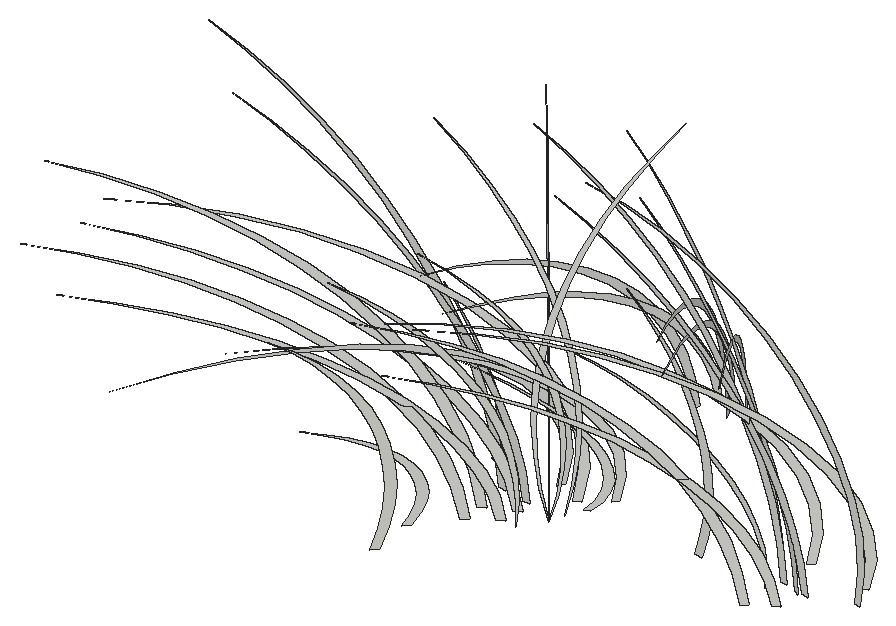
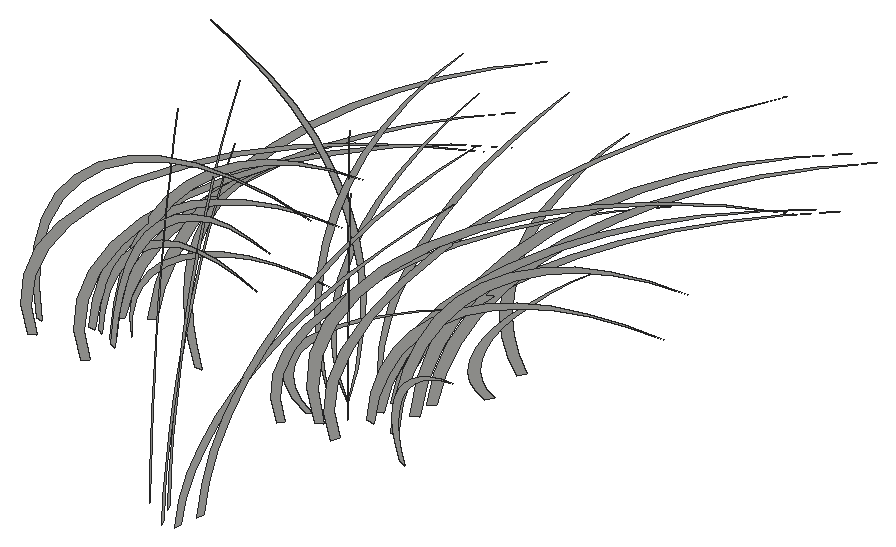
# SketchUp Ruby script. Lengths in inches.
U = 1.inch
M = Sketchup.active_model
def pt(a) = Geom::Point3d.new(a.map { |v| v * U })
def face(e, loops, mat)
  f = e.add_face(loops[0].map { |a| pt(a) })
  loops[1..].each { |l| e.add_face(l.map { |a| pt(a) }).erase! }
  f.material = f.back_material = mat if mat
  f
end
# faces: each face lists its corners as indices into pts; further lists are holes
def faces(e, pts, list, mat = nil) = list.each { |f| face(e, (f[0].is_a?(Array) ? f : [f]).map { |l| l.map { |i| pts[i] } }, mat) }
# xy, xz, yz: faces in a plane at the given z, y or x. An outline is a flat list of corners, or four numbers for a rectangle; further outlines are holes
def ring(l) = l.size == 4 ? [[l[0], l[1]], [l[2], l[1]], [l[2], l[3]], [l[0], l[3]]] : l.each_slice(2).to_a
def flat(e, list, mat, &to3) = list.each { |f| face(e, (f[0].is_a?(Array) ? f : [f]).map { |l| ring(l).map { |u, v| to3.(u, v) } }, mat) }
def xy(e, z, list, mat = nil) = flat(e, list, mat) { |x, y| [x, y, z] }
def xz(e, y, list, mat = nil) = flat(e, list, mat) { |x, z| [x, y, z] }
def yz(e, x, list, mat = nil) = flat(e, list, mat) { |y, z| [x, y, z] }
def lines(e, pts, list) = list.each { |a, b| e.add_line(pt(pts[a]), pt(pts[b])) }
# prism: a flat outline (further loops are holes) pulled along v
def prism(e, loops, v, mat = nil)
  f = face(e, loops, mat); d = Geom::Vector3d.new(v.map { |x| x * U })
  f.pushpull(f.normal.samedirection?(d) ? d.length : -d.length)
end
def box(e, o, s, mat = nil) = prism(e, [[o, [o[0] + s[0], o[1], o[2]], [o[0] + s[0], o[1] + s[1], o[2]], [o[0], o[1] + s[1], o[2]]]], [0, 0, s[2]], mat)
def at(x, y, z, deg = 0) = Geom::Transformation.translation(pt([x, y, z])) * Geom::Transformation.rotation(ORIGIN, Z_AXIS, deg.degrees)
def axes(o, x, y, z) = Geom::Transformation.new([*x, 0, *y, 0, *z, 0, *pt(o).to_a, 1])
def part(name) = M.definitions.add(name)
# library, detail: a bought-in or finely detailed component or shape, given as its bounding box
def library(name, o, s) = part(name).tap { |d| box(d.entities, o, s) }
def detail(e, o, s) = box(e.add_group.entities, o, s)
def put(e, d, t, mat = nil) = e.add_instance(d, t).tap { |i| i.material = mat if mat }
def group(e, t, mat = nil) = e.add_group.tap { |g| g.transformation = t; g.material = mat if mat }.entities
root = M.entities
g1 = group(root,at(60.55,564.61,0.02))
p = [[-20.46,3.64,18.05],[-23.54,4.19,18.53],[-20.55,3.66,17.95],[-17.67,3.15,17.15],[-14.91,2.66,16.14],[-12.33,2.2,14.93],
  [-9.93,1.77,13.53],[-7.76,1.38,11.96],[-5.84,1.04,10.23],[-4.18,0.74,8.37],[-2.8,0.5,6.39],[-1.73,0.31,4.32],
  [-0.97,0.17,2.18],[-0.53,0.09,0],[0,0,0],[-0.36,0.0625,2.23],[-1.07,0.19,4.43],[-2.125,0.38,6.55],
  [-3.51,0.625,8.57],[-5.2,0.93,10.47],[-7.1875,1.28,12.22],[-9.43,1.68,13.8],[-11.92,2.125,15.1875],[-14.61,2.6,16.37],
  [-17.46,3.11,17.33]]
faces(g1,p,[[0,1,2,3,4,5,6,7,8,9,10,11,12,13,14,15,16,17,18,19,20,21,22,23,24]])
g2 = group(root,at(60.9375,562.5,0.02))
p = [[-18.45,-9.5625,18.05],[-21.23,-11,18.53],[-18.53,-9.61,17.95],[-15.93,-8.26,17.15],[-13.45,-6.97,16.14],[-11.12,-5.76,14.93],
  [-8.96,-4.64,13.53],[-7,-3.63,11.96],[-5.26,-2.73,10.23],[-3.77,-1.95,8.37],[-2.53,-1.3125,6.39],[-1.5625,-0.81,4.32],
  [-0.875,-0.45,2.18],[-0.48,-0.25,0],[0,0,0],[-0.32,-0.17,2.23],[-0.97,-0.5,4.43],[-1.92,-0.99,6.55],
  [-3.16,-1.64,8.57],[-4.69,-2.43,10.47],[-6.48,-3.36,12.22],[-8.51,-4.41,13.8],[-10.75,-5.57,15.1875],[-13.17,-6.83,16.37],
  [-15.75,-8.16,17.33]]
faces(g2,p,[[0,1,2,3,4,5,6,7,8,9,10,11,12,13,14,15,16,17,18,19,20,21,22,23,24]])
g3 = group(root,at(60.9375,562.5,0.02))
p = [[-18.45,-9.5625,18.05],[-21.23,-11,18.53],[-18.53,-9.61,17.95],[-15.93,-8.26,17.15],[-13.45,-6.97,16.14],[-11.12,-5.76,14.93],
  [-8.96,-4.64,13.53],[-7,-3.63,11.96],[-5.26,-2.73,10.23],[-3.77,-1.95,8.37],[-2.53,-1.3125,6.39],[-1.5625,-0.81,4.32],
  [-0.875,-0.45,2.18],[-0.48,-0.25,0],[0,0,0],[-0.32,-0.17,2.23],[-0.97,-0.5,4.43],[-1.92,-0.99,6.55],
  [-3.16,-1.64,8.57],[-4.69,-2.43,10.47],[-6.48,-3.36,12.22],[-8.51,-4.41,13.8],[-10.75,-5.57,15.1875],[-13.17,-6.83,16.37],
  [-15.75,-8.16,17.33]]
faces(g3,p,[[0,1,2,3,4,5,6,7,8,9,10,11,12,13,14,15,16,17,18,19,20,21,22,23,24]])
g4 = group(root,at(62.45,564.27,0.02))
p = [[-20.46,3.64,14.56],[-23.54,4.19,14.94],[-20.55,3.66,14.48],[-17.67,3.15,13.83],[-14.91,2.66,13.02],[-12.33,2.2,12.04],
  [-9.93,1.77,10.91],[-7.76,1.38,9.64],[-5.84,1.04,8.25],[-4.18,0.74,6.75],[-2.8,0.5,5.15],[-1.73,0.31,3.49],
  [-0.97,0.17,1.76],[-0.53,0.09,0],[0,0,0],[-0.36,0.0625,1.8],[-1.07,0.19,3.57],[-2.125,0.38,5.28],
  [-3.51,0.625,6.91],[-5.2,0.93,8.44],[-7.1875,1.28,9.85],[-9.43,1.68,11.13],[-11.92,2.125,12.25],[-14.61,2.6,13.2],
  [-17.46,3.11,13.97]]
faces(g4,p,[[0,1,2,3,4,5,6,7,8,9,10,11,12,13,14,15,16,17,18,19,20,21,22,23,24]])
g5 = group(root,at(60.98,561.01,0.02))
p = [[-17.17,-11.7,15.34],[-19.76,-13.47,15.75],[-17.25,-11.76,15.26],[-14.83,-10.11,14.58],[-12.52,-8.53,13.72],[-10.35,-7.05,12.69],
  [-8.34,-5.68,11.5],[-6.52,-4.44,10.16],[-4.9,-3.34,8.7],[-3.51,-2.39,7.11],[-2.35,-1.6,5.43],[-1.45,-0.99,3.67],
  [-0.82,-0.56,1.86],[-0.45,-0.3,0],[0,0,0],[-0.3,-0.21,1.9],[-0.9,-0.61,3.76],[-1.78,-1.22,5.57],
  [-2.95,-2.01,7.28],[-4.37,-2.98,8.9],[-6.03,-4.11,10.39],[-7.92,-5.4,11.73],[-10,-6.82,12.91],[-12.26,-8.36,13.91],
  [-14.66,-9.99,14.73]]
faces(g5,p,[[0,1,2,3,4,5,6,7,8,9,10,11,12,13,14,15,16,17,18,19,20,21,22,23,24]])
g6 = group(root,at(62.65,563.39,0.02))
p = [[-18.45,-9.5625,14.56],[-21.23,-11,14.94],[-18.53,-9.61,14.48],[-15.93,-8.26,13.83],[-13.45,-6.97,13.02],[-11.12,-5.76,12.04],
  [-8.96,-4.64,10.91],[-7,-3.63,9.64],[-5.26,-2.73,8.25],[-3.77,-1.95,6.75],[-2.53,-1.3125,5.15],[-1.5625,-0.81,3.49],
  [-0.875,-0.45,1.76],[-0.48,-0.25,0],[0,0,0],[-0.32,-0.17,1.8],[-0.97,-0.5,3.57],[-1.92,-0.99,5.28],
  [-3.16,-1.64,6.91],[-4.69,-2.43,8.44],[-6.48,-3.36,9.85],[-8.51,-4.41,11.13],[-10.75,-5.57,12.25],[-13.17,-6.83,13.2],
  [-15.75,-8.16,13.97]]
faces(g6,p,[[0,1,2,3,4,5,6,7,8,9,10,11,12,13,14,15,16,17,18,19,20,21,22,23,24]])
g7 = group(root,at(62.65,563.39,0.02))
p = [[-18.45,-9.5625,14.56],[-21.23,-11,14.94],[-18.53,-9.61,14.48],[-15.93,-8.26,13.83],[-13.45,-6.97,13.02],[-11.12,-5.76,12.04],
  [-8.96,-4.64,10.91],[-7,-3.63,9.64],[-5.26,-2.73,8.25],[-3.77,-1.95,6.75],[-2.53,-1.3125,5.15],[-1.5625,-0.81,3.49],
  [-0.875,-0.45,1.76],[-0.48,-0.25,0],[0,0,0],[-0.32,-0.17,1.8],[-0.97,-0.5,3.57],[-1.92,-0.99,5.28],
  [-3.16,-1.64,6.91],[-4.69,-2.43,8.44],[-6.48,-3.36,9.85],[-8.51,-4.41,11.13],[-10.75,-5.57,12.25],[-13.17,-6.83,13.2],
  [-15.75,-8.16,13.97]]
faces(g7,p,[[0,1,2,3,4,5,6,7,8,9,10,11,12,13,14,15,16,17,18,19,20,21,22,23,24]])
g8 = group(root,at(62.58,562.1,0.02))
p = [[-17.17,-11.7,12.375],[-19.76,-13.47,12.7],[-17.25,-11.76,12.31],[-14.83,-10.11,11.76],[-12.52,-8.53,11.07],[-10.35,-7.05,10.23],
  [-8.34,-5.68,9.27],[-6.52,-4.44,8.2],[-4.9,-3.34,7.01],[-3.51,-2.39,5.74],[-2.35,-1.6,4.38],[-1.45,-0.99,2.96],
  [-0.82,-0.56,1.5],[-0.45,-0.3,0],[0,0,0],[-0.3,-0.21,1.53],[-0.9,-0.61,3.03],[-1.78,-1.22,4.49],
  [-2.95,-2.01,5.875],[-4.37,-2.98,7.18],[-6.03,-4.11,8.375],[-7.92,-5.4,9.46],[-10,-6.82,10.41],[-12.26,-8.36,11.22],
  [-14.66,-9.99,11.88]]
faces(g8,p,[[0,1,2,3,4,5,6,7,8,9,10,11,12,13,14,15,16,17,18,19,20,21,22,23,24]])
g9 = group(root,at(64.78,566.42,0.02))
p = [[-0.82,-0.43,0],[-0.36,-0.1875,0],[0,0,2.0625],[-0.15,-0.08,4.13],[-0.8,-0.42,6.16],[-1.95,-1.01,8.1],
  [-3.57,-1.85,9.91],[-5.6,-2.9,11.52],[-8.01,-4.15,12.92],[-10.74,-5.57,14.05],[-13.71,-7.1,14.9],[-16.85,-8.73,15.45],
  [-20.09,-10.41,15.67],[-23.34,-12.1,15.5625],[-20.15,-10.44,15.58],[-16.99,-8.81,15.29],[-13.9375,-7.22,14.71],[-11.06,-5.73,13.83],
  [-8.42,-4.37,12.68],[-6.09,-3.16,11.3],[-4.11,-2.13,9.7],[-2.53,-1.3125,7.9375],[-1.4,-0.72,6.04],[-0.72,-0.375,4.05],
  [-0.53,-0.27,2.02]]
faces(g9,p,[[0,1,2,3,4,5,6,7,8,9,10,11,12,13,14,15,16,17,18,19,20,21,22,23,24]])
g10 = group(root,at(59.1,566.3,0.02))
p = [[-6.53,2.99,7.88],[-5.33,2.44,7.38],[-4.26,1.95,6.83],[-3.3,1.51,6.24],[-2.48,1.14,5.62],[-1.81,0.83,4.96],
  [-1.28,0.58,4.27],[-0.9,0.41,3.57],[-0.68,0.31,2.86],[-0.61,0.28,2.13],[-0.71,0.32,1.41],[-0.96,0.4375,0.7],
  [-1.37,0.625,0],[-0.84,0.38,0],[-0.39,0.18,0.71],[-0.11,0.05,1.43],[0,0,2.17],[-0.07,0.03,2.9],
  [-0.32,0.15,3.63],[-0.74,0.34,4.34],[-1.33,0.61,5.03],[-2.08,0.95,5.69],[-2.99,1.37,6.3125],[-4.04,1.85,6.89],
  [-5.22,2.39,7.41]]
faces(g10,p,[[0,1,2,3,4,5,6,7,8,9,10,11,12,13,14,15,16,17,18,19,20,21,22,23,24]])
g11 = group(root,at(62.69,567.61,0.02))
p = [[-0.37,-0.92,0],[-0.16,-0.41,0],[0,0,1.75],[-0.07,-0.17,3.51],[-0.36,-0.9,5.24],[-0.88,-2.19,6.89],
  [-1.61,-4,8.42],[-2.53,-6.28,9.8],[-3.61,-8.99,10.98],[-4.84,-12.04,11.95],[-6.18,-15.375,12.67],[-7.6,-18.9,13.13],
  [-9.06,-22.53,13.32],[-10.53,-26.18,13.23],[-9.09,-22.6,13.25],[-7.66,-19.06,13],[-6.29,-15.63,12.5],[-4.99,-12.41,11.75],
  [-3.8,-9.45,10.78],[-2.75,-6.83,9.6],[-1.85,-4.61,8.25],[-1.14,-2.84,6.75],[-0.63,-1.57,5.13],[-0.33,-0.8125,3.44],
  [-0.24,-0.59,1.72]]
faces(g11,p,[[0,1,2,3,4,5,6,7,8,9,10,11,12,13,14,15,16,17,18,19,20,21,22,23,24]])
g12 = group(root,at(59.4375,559.42,0.02))
p = [[-3.94,-6,6.7],[-3.22,-4.9,6.27],[-2.57,-3.91,5.81],[-2,-3.04,5.31],[-1.5,-2.28,4.77],[-1.09,-1.66,4.21],
  [-0.77,-1.17,3.63],[-0.54,-0.83,3.03],[-0.41,-0.62,2.43],[-0.37,-0.5625,1.8125],[-0.43,-0.65,1.2],[-0.58,-0.88,0.59],
  [-0.83,-1.26,0],[-0.51,-0.77,0],[-0.23,-0.36,0.6],[-0.0625,-0.1,1.22],[0,0,1.84],[-0.04,-0.07,2.47],
  [-0.19,-0.29,3.09],[-0.45,-0.68,3.69],[-0.8,-1.22,4.28],[-1.26,-1.91,4.84],[-1.81,-2.75,5.37],[-2.44,-3.71,5.86],
  [-3.16,-4.8,6.3]]
faces(g12,p,[[0,1,2,3,4,5,6,7,8,9,10,11,12,13,14,15,16,17,18,19,20,21,22,23,24]])
g13 = group(root,at(59.73,556.34,0.02))
p = [[-3.94,-6,13.62],[-3.22,-4.9,12.76],[-2.57,-3.91,11.81],[-2,-3.04,10.79],[-1.5,-2.28,9.7],[-1.09,-1.66,8.57],
  [-0.77,-1.17,7.38],[-0.54,-0.83,6.17],[-0.41,-0.62,4.93],[-0.37,-0.5625,3.6875],[-0.43,-0.65,2.44],[-0.58,-0.88,1.21],
  [-0.83,-1.26,0],[-0.51,-0.77,0],[-0.23,-0.36,1.22],[-0.0625,-0.1,2.48],[0,0,3.75],[-0.04,-0.07,5.02],
  [-0.19,-0.29,6.28],[-0.45,-0.68,7.51],[-0.8,-1.22,8.7],[-1.26,-1.91,9.84],[-1.81,-2.75,10.91],[-2.44,-3.71,11.9],
  [-3.16,-4.8,12.8125]]
faces(g13,p,[[0,1,2,3,4,5,6,7,8,9,10,11,12,13,14,15,16,17,18,19,20,21,22,23,24]])
g14 = group(root,at(66.2,567.76,0.02))
p = [[-0.5,-0.57,0],[-0.22,-0.25,0],[0,0,1.46],[-0.09,-0.1,2.93],[-0.49,-0.56,4.375],[-1.19,-1.35,5.75],
  [-2.17,-2.47,7.03],[-3.41,-3.89,8.18],[-4.88,-5.56,9.17],[-6.54,-7.45,9.98],[-8.36,-9.51,10.58],[-10.27,-11.69,10.97],
  [-12.24,-13.9375,11.125],[-14.23,-16.19,11.05],[-12.28,-13.98,11.0625],[-10.36,-11.79,10.86],[-8.5,-9.67,10.44],[-6.74,-7.67,9.82],
  [-5.13,-5.84,9.01],[-3.71,-4.22,8.02],[-2.51,-2.85,6.89],[-1.54,-1.76,5.64],[-0.85,-0.97,4.29],[-0.44,-0.5,2.88],
  [-0.32,-0.37,1.4375]]
faces(g14,p,[[0,1,2,3,4,5,6,7,8,9,10,11,12,13,14,15,16,17,18,19,20,21,22,23,24]])
g15 = group(root,at(66.2,567.76,0.02))
p = [[-0.5,-0.57,0],[-0.22,-0.25,0],[0,0,1.46],[-0.09,-0.1,2.93],[-0.49,-0.56,4.375],[-1.19,-1.35,5.75],
  [-2.17,-2.47,7.03],[-3.41,-3.89,8.18],[-4.88,-5.56,9.17],[-6.54,-7.45,9.98],[-8.36,-9.51,10.58],[-10.27,-11.69,10.97],
  [-12.24,-13.9375,11.125],[-14.23,-16.19,11.05],[-12.28,-13.98,11.0625],[-10.36,-11.79,10.86],[-8.5,-9.67,10.44],[-6.74,-7.67,9.82],
  [-5.13,-5.84,9.01],[-3.71,-4.22,8.02],[-2.51,-2.85,6.89],[-1.54,-1.76,5.64],[-0.85,-0.97,4.29],[-0.44,-0.5,2.88],
  [-0.32,-0.37,1.4375]]
faces(g15,p,[[0,1,2,3,4,5,6,7,8,9,10,11,12,13,14,15,16,17,18,19,20,21,22,23,24]])
g16 = group(root,at(63.3125,564.77,0.02))
p = [[-6.74,8.21,19.61],[-5.67,6.9,18.16],[-4.68,5.7,16.67],[-3.78,4.6,15.125],[-2.98,3.62,13.55],[-2.27,2.76,11.93],
  [-1.65,2.01,10.28],[-1.14,1.39,8.61],[-0.72,0.88,6.91],[-0.41,0.5,5.2],[-0.2,0.24,3.47],[-0.09,0.11,1.74],
  [-0.09,0.11,0],[0,0,1.74],[-0.03,0.04,3.49],[-0.1875,0.23,5.23],[-0.46,0.56,6.96],[-0.85,1.04,8.67],
  [-1.36,1.66,10.36],[-1.98,2.42,12.01],[-2.72,3.3125,13.63],[-3.57,4.35,15.21],[-4.52,5.51,16.73],[-5.58,6.8,18.2]]
faces(g16,p,[[0,1,2,3,4,5,6,7,8,9,10,11,12,13,14,15,16,17,18,19,20,21,22,23]])
g17 = group(root,at(63.3125,564.77,0.02))
p = [[-6.74,8.21,19.61],[-5.67,6.9,18.16],[-4.68,5.7,16.67],[-3.78,4.6,15.125],[-2.98,3.62,13.55],[-2.27,2.76,11.93],
  [-1.65,2.01,10.28],[-1.14,1.39,8.61],[-0.72,0.88,6.91],[-0.41,0.5,5.2],[-0.2,0.24,3.47],[-0.09,0.11,1.74],
  [-0.09,0.11,0],[0,0,1.74],[-0.03,0.04,3.49],[-0.1875,0.23,5.23],[-0.46,0.56,6.96],[-0.85,1.04,8.67],
  [-1.36,1.66,10.36],[-1.98,2.42,12.01],[-2.72,3.3125,13.63],[-3.57,4.35,15.21],[-4.52,5.51,16.73],[-5.58,6.8,18.2]]
faces(g17,p,[[0,1,2,3,4,5,6,7,8,9,10,11,12,13,14,15,16,17,18,19,20,21,22,23]])
g18 = group(root,at(63.46,562.02,0.02))
p = [[-5.83,-8.875,16.67],[-4.9,-7.46,15.44],[-4.05,-6.16,14.17],[-3.27,-4.98,12.86],[-2.58,-3.92,11.51],[-1.96,-2.98,10.14],
  [-1.43,-2.18,8.74],[-0.99,-1.5,7.31],[-0.63,-0.95,5.87],[-0.36,-0.54,4.42],[-0.17,-0.26,2.95],[-0.08,-0.12,1.48],
  [-0.08,-0.12,0],[0,0,1.48],[-0.03,-0.04,2.97],[-0.16,-0.24,4.45],[-0.4,-0.6,5.92],[-0.74,-1.12,7.37],
  [-1.18,-1.79,8.81],[-1.72,-2.61,10.21],[-2.36,-3.58,11.59],[-3.09,-4.7,12.93],[-3.92,-5.96,14.22],[-4.83,-7.35,15.47]]
faces(g18,p,[[0,1,2,3,4,5,6,7,8,9,10,11,12,13,14,15,16,17,18,19,20,21,22,23]])
g19 = group(root,at(62.85,578.16,0.02))
p = [[-3,-16.83,14.86],[-3.45,-19.375,15.25],[-3.01,-16.91,14.77],[-2.59,-14.54,14.12],[-2.1875,-12.27,13.29],[-1.81,-10.14,12.29],
  [-1.46,-8.18,11.14],[-1.14,-6.39,9.84],[-0.86,-4.8,8.42],[-0.61,-3.4375,6.89],[-0.41,-2.31,5.26],[-0.25,-1.42,3.56],
  [-0.14,-0.8,1.8],[-0.08,-0.4375,0],[0,0,0],[-0.05,-0.3,1.84],[-0.16,-0.88,3.64],[-0.3125,-1.75,5.39],
  [-0.51,-2.89,7.05],[-0.76,-4.28,8.62],[-1.05,-5.91,10.06],[-1.38,-7.76,11.36],[-1.75,-9.81,12.5],[-2.14,-12.02,13.47],
  [-2.56,-14.375,14.26]]
faces(g19,p,[[0,1,2,3,4,5,6,7,8,9,10,11,12,13,14,15,16,17,18,19,20,21,22,23,24]])
g20 = group(root,at(63.13,579.73,0.02))
p = [[-3,-16.83,11.98],[-3.45,-19.375,12.3],[-3.01,-16.91,11.91],[-2.59,-14.54,11.39],[-2.1875,-12.27,10.71],[-1.81,-10.14,9.91],
  [-1.46,-8.18,8.98],[-1.14,-6.39,7.9375],[-0.86,-4.8,6.79],[-0.61,-3.4375,5.55],[-0.41,-2.31,4.24],[-0.25,-1.42,2.87],
  [-0.14,-0.8,1.45],[-0.08,-0.4375,0],[0,0,0],[-0.05,-0.3,1.48],[-0.16,-0.88,2.9375],[-0.3125,-1.75,4.35],
  [-0.51,-2.89,5.6875],[-0.76,-4.28,6.95],[-1.05,-5.91,8.11],[-1.38,-7.76,9.16],[-1.75,-9.81,10.08],[-2.14,-12.02,10.87],
  [-2.56,-14.375,11.5]]
faces(g20,p,[[0,1,2,3,4,5,6,7,8,9,10,11,12,13,14,15,16,17,18,19,20,21,22,23,24]])
g21 = group(root,at(65.5625,564.74,0.02))
p = [[-0.89,-0.32,0],[-0.4,-0.14,1.97],[-0.1,-0.04,3.96],[0,0,5.95],[-0.1,-0.03,7.95],[-0.39,-0.14,9.9375],
  [-0.89,-0.3125,11.91],[-1.57,-0.56,13.85],[-2.45,-0.87,15.76],[-3.52,-1.25,17.63],[-4.77,-1.6875,19.44],[-6.19,-2.19,21.2],
  [-7.79,-2.76,22.89],[-6.29,-2.23,21.17],[-4.94,-1.75,19.4],[-3.76,-1.33,17.58],[-2.74,-0.97,15.71],[-1.89,-0.67,13.8],
  [-1.22,-0.43,11.86],[-0.72,-0.25,9.9],[-0.4,-0.14,7.93],[-0.25,-0.09,5.94],[-0.29,-0.1,3.95],[-0.5,-0.18,1.97]]
faces(g21,p,[[0,1,2,3,4,5,6,7,8,9,10,11,12,13,14,15,16,17,18,19,20,21,22,23]])
g22 = group(root,at(66.66,566.1,0.02))
p = [[-9.01,-2.98,7.88],[-7.3,-2.41,7.38],[-5.75,-1.9,6.83],[-4.38,-1.45,6.24],[-3.2,-1.06,5.62],[-2.23,-0.74,4.96],
  [-1.47,-0.49,4.27],[-0.92,-0.31,3.57],[-0.61,-0.2,2.86],[-0.51,-0.17,2.13],[-0.65,-0.21,1.41],[-1.01,-0.33,0.7],
  [-1.6,-0.53,0],[-1.21,-0.4,0],[-0.54,-0.18,0.69],[-0.12,-0.04,1.4],[0.06,0.02,2.13],[-0.02,-0.01,2.85],
  [-0.35,-0.11,3.58],[-0.92,-0.3,4.29],[-1.73,-0.57,4.98],[-2.78,-0.92,5.64],[-4.05,-1.34,6.27],[-5.52,-1.82,6.86],
  [-7.18,-2.375,7.4]]
faces(g22,p,[[0,1,2,3,4,5,6,7,8,9,10,11,12,13,14,15,16,17,18,19,20,21,22,23,24]])
g23 = group(root,at(65,562.72,0.02))
p = [[-0.6,0.73,0],[-0.27,0.33,1.77],[-0.07,0.08,3.57],[0,0,5.36],[-0.07,0.08,7.16],[-0.27,0.32,8.95],
  [-0.6,0.73,10.73],[-1.06,1.29,12.48],[-1.65,2.01,14.2],[-2.37,2.88,15.88],[-3.21,3.91,17.52],[-4.17,5.08,19.1],
  [-5.25,6.39,20.625],[-4.23,5.15,19.08],[-3.33,4.05,17.48],[-2.53,3.08,15.83],[-1.84,2.25,14.15],[-1.27,1.55,12.43],
  [-0.82,1,10.6875],[-0.48,0.59,8.92],[-0.27,0.32,7.14],[-0.17,0.21,5.35],[-0.19,0.24,3.5625],[-0.34,0.41,1.78]]
faces(g23,p,[[0,1,2,3,4,5,6,7,8,9,10,11,12,13,14,15,16,17,18,19,20,21,22,23]])
g24 = group(root,at(64.92,564.24,0.02))
p = [[-0.52,-0.79,0],[-0.23,-0.35,1.51],[-0.06,-0.09,3.03],[0,0,4.56],[-0.06,-0.09,6.09],[-0.23,-0.35,7.61],
  [-0.52,-0.79,9.12],[-0.92,-1.39,10.61],[-1.43,-2.17,12.07],[-2.05,-3.12,13.5],[-2.78,-4.23,14.89],[-3.61,-5.49,16.24],
  [-4.54,-6.91,17.53],[-3.66,-5.57,16.21],[-2.88,-4.38,14.86],[-2.1875,-3.33,13.46],[-1.6,-2.43,12.03],[-1.1,-1.68,10.57],
  [-0.71,-1.08,9.08],[-0.42,-0.64,7.58],[-0.23,-0.35,6.07],[-0.15,-0.22,4.55],[-0.17,-0.25,3.03],[-0.29,-0.44,1.51]]
faces(g24,p,[[0,1,2,3,4,5,6,7,8,9,10,11,12,13,14,15,16,17,18,19,20,21,22,23]])
g25 = group(root,at(63.73,562.78,0.02))
p = [[0.67,0.67,0],[0.3,0.3,2.04],[0.08,0.08,4.1],[0,0,6.17],[0.07,0.07,8.23],[0.3,0.3,10.29],
  [0.66,0.66,12.33],[1.18,1.18,14.34],[1.84,1.84,16.32],[2.64,2.64,18.26],[3.58,3.58,20.14],[4.65,4.65,21.96],
  [5.84,5.84,23.71],[4.72,4.72,21.93],[3.71,3.71,20.09],[2.82,2.82,18.2],[2.05,2.05,16.26],[1.42,1.42,14.29],
  [0.91,0.91,12.29],[0.54,0.54,10.26],[0.3,0.3,8.21],[0.1875,0.1875,6.15],[0.22,0.22,4.09],[0.375,0.375,2.04]]
faces(g25,p,[[0,1,2,3,4,5,6,7,8,9,10,11,12,13,14,15,16,17,18,19,20,21,22,23]])
g26 = group(root,at(78.56,565.95,0.02))
p = [[-17.99,3.82,18.36],[-20.7,4.4,18.85],[-18.07,3.84,18.26],[-15.53,3.3,17.45],[-13.11,2.79,16.42],[-10.84,2.3,15.1875],
  [-8.73,1.86,13.76],[-6.83,1.45,12.16],[-5.13,1.09,10.41],[-3.67,0.78,8.51],[-2.47,0.52,6.5],[-1.52,0.32,4.4],
  [-0.85,0.18,2.22],[-0.47,0.1,0],[0,0,0],[-0.32,0.07,2.27],[-0.94,0.2,4.5],[-1.87,0.4,6.66],
  [-3.09,0.66,8.72],[-4.57,0.97,10.65],[-6.32,1.34,12.43],[-8.3,1.76,14.04],[-10.48,2.23,15.45],[-12.84,2.73,16.65],
  [-15.36,3.26,17.625]]
faces(g26,p,[[0,1,2,3,4,5,6,7,8,9,10,11,12,13,14,15,16,17,18,19,20,21,22,23,24]])
g27 = group(root,at(63.85,579.89,0.02))
p = [[7.87,-15.18,11.98],[9.06,-17.47,12.3],[7.91,-15.25,11.91],[6.8,-13.11,11.39],[5.74,-11.07,10.71],[4.74,-9.15,9.91],
  [3.82,-7.37,8.98],[2.99,-5.76,7.9375],[2.25,-4.33,6.79],[1.61,-3.1,5.55],[1.08,-2.08,4.24],[0.67,-1.28,2.87],
  [0.375,-0.72,1.45],[0.21,-0.4,0],[0,0,0],[0.14,-0.27,1.48],[0.41,-0.8,2.9375],[0.82,-1.58,4.35],
  [1.35,-2.6,5.6875],[2,-3.86,6.95],[2.76,-5.33,8.11],[3.63,-7,9.16],[4.59,-8.85,10.08],[5.62,-10.84,10.87],
  [6.72,-12.96,11.5]]
faces(g27,p,[[0,1,2,3,4,5,6,7,8,9,10,11,12,13,14,15,16,17,18,19,20,21,22,23,24]])
g28 = group(root,at(63.85,579.89,0.02))
p = [[7.87,-15.18,11.98],[9.06,-17.47,12.3],[7.91,-15.25,11.91],[6.8,-13.11,11.39],[5.74,-11.07,10.71],[4.74,-9.15,9.91],
  [3.82,-7.37,8.98],[2.99,-5.76,7.9375],[2.25,-4.33,6.79],[1.61,-3.1,5.55],[1.08,-2.08,4.24],[0.67,-1.28,2.87],
  [0.375,-0.72,1.45],[0.21,-0.4,0],[0,0,0],[0.14,-0.27,1.48],[0.41,-0.8,2.9375],[0.82,-1.58,4.35],
  [1.35,-2.6,5.6875],[2,-3.86,6.95],[2.76,-5.33,8.11],[3.63,-7,9.16],[4.59,-8.85,10.08],[5.62,-10.84,10.87],
  [6.72,-12.96,11.5]]
faces(g28,p,[[0,1,2,3,4,5,6,7,8,9,10,11,12,13,14,15,16,17,18,19,20,21,22,23,24]])
g29 = group(root,at(78.15,566.33,0.02))
p = [[-16.23,8.63,15.97],[-18.68,9.93,16.4],[-16.3125,8.67,15.89],[-14.02,7.45,15.18],[-11.84,6.29,14.29],[-9.78,5.2,13.21],
  [-7.88,4.19,11.97],[-6.16,3.28,10.58],[-4.63,2.46,9.05],[-3.32,1.76,7.41],[-2.23,1.18,5.66],[-1.375,0.73,3.82],
  [-0.77,0.41,1.93],[-0.42,0.22,0],[0,0,0],[-0.29,0.15,1.98],[-0.85,0.45,3.92],[-1.6875,0.9,5.79],
  [-2.78,1.48,7.58],[-4.13,2.2,9.26],[-5.7,3.03,10.8125],[-7.49,3.98,12.21],[-9.46,5.03,13.44],[-11.59,6.16,14.49],
  [-13.86,7.37,15.33]]
faces(g29,p,[[0,1,2,3,4,5,6,7,8,9,10,11,12,13,14,15,16,17,18,19,20,21,22,23,24]])
g30 = group(root,at(78.62,568.9,0.02))
p = [[-0.67,-0.47,0],[-0.3,-0.21,0],[0,0,1.82],[-0.12,-0.08,3.66],[-0.66,-0.46,5.45],[-1.6,-1.11,7.17],
  [-2.91,-2.03,8.77],[-4.58,-3.19,10.2],[-6.55,-4.57,11.43],[-8.78,-6.12,12.4375],[-11.2,-7.82,13.1875],[-13.77,-9.61,13.67],
  [-16.42,-11.46,13.87],[-19.08,-13.31,13.77],[-16.47,-11.49,13.79],[-13.89,-9.6875,13.54],[-11.39,-7.95,13.01],[-9.04,-6.31,12.24],
  [-6.88,-4.8,11.22],[-4.98,-3.47,10],[-3.36,-2.34,8.59],[-2.07,-1.44,7.02],[-1.14,-0.8,5.34],[-0.59,-0.41,3.59],
  [-0.43,-0.3,1.79]]
faces(g30,p,[[0,1,2,3,4,5,6,7,8,9,10,11,12,13,14,15,16,17,18,19,20,21,22,23,24]])
g31 = group(root,at(78.62,568.9,0.02))
p = [[-0.67,-0.47,0],[-0.3,-0.21,0],[0,0,1.82],[-0.12,-0.08,3.66],[-0.66,-0.46,5.45],[-1.6,-1.11,7.17],
  [-2.91,-2.03,8.77],[-4.58,-3.19,10.2],[-6.55,-4.57,11.43],[-8.78,-6.12,12.4375],[-11.2,-7.82,13.1875],[-13.77,-9.61,13.67],
  [-16.42,-11.46,13.87],[-19.08,-13.31,13.77],[-16.47,-11.49,13.79],[-13.89,-9.6875,13.54],[-11.39,-7.95,13.01],[-9.04,-6.31,12.24],
  [-6.88,-4.8,11.22],[-4.98,-3.47,10],[-3.36,-2.34,8.59],[-2.07,-1.44,7.02],[-1.14,-0.8,5.34],[-0.59,-0.41,3.59],
  [-0.43,-0.3,1.79]]
faces(g31,p,[[0,1,2,3,4,5,6,7,8,9,10,11,12,13,14,15,16,17,18,19,20,21,22,23,24]])
g32 = group(root,at(64.58,578.48,0.02))
p = [[7.87,-15.18,14.86],[9.06,-17.47,15.25],[7.91,-15.25,14.77],[6.8,-13.11,14.12],[5.74,-11.07,13.29],[4.74,-9.15,12.29],
  [3.82,-7.37,11.14],[2.99,-5.76,9.84],[2.25,-4.33,8.42],[1.61,-3.1,6.89],[1.08,-2.08,5.26],[0.67,-1.28,3.56],
  [0.375,-0.72,1.8],[0.21,-0.4,0],[0,0,0],[0.14,-0.27,1.84],[0.41,-0.8,3.64],[0.82,-1.58,5.39],
  [1.35,-2.6,7.05],[2,-3.86,8.62],[2.76,-5.33,10.06],[3.63,-7,11.36],[4.59,-8.85,12.5],[5.62,-10.84,13.47],
  [6.72,-12.96,14.26]]
faces(g32,p,[[0,1,2,3,4,5,6,7,8,9,10,11,12,13,14,15,16,17,18,19,20,21,22,23,24]])
g33 = group(root,at(64.58,578.48,0.02))
p = [[7.87,-15.18,14.86],[9.06,-17.47,15.25],[7.91,-15.25,14.77],[6.8,-13.11,14.12],[5.74,-11.07,13.29],[4.74,-9.15,12.29],
  [3.82,-7.37,11.14],[2.99,-5.76,9.84],[2.25,-4.33,8.42],[1.61,-3.1,6.89],[1.08,-2.08,5.26],[0.67,-1.28,3.56],
  [0.375,-0.72,1.8],[0.21,-0.4,0],[0,0,0],[0.14,-0.27,1.84],[0.41,-0.8,3.64],[0.82,-1.58,5.39],
  [1.35,-2.6,7.05],[2,-3.86,8.62],[2.76,-5.33,10.06],[3.63,-7,11.36],[4.59,-8.85,12.5],[5.62,-10.84,13.47],
  [6.72,-12.96,14.26]]
faces(g33,p,[[0,1,2,3,4,5,6,7,8,9,10,11,12,13,14,15,16,17,18,19,20,21,22,23,24]])
g34 = group(root,at(78.33,562.97,0.02))
p = [[-15.08,-10.52,15.97],[-17.36,-12.11,16.4],[-15.15,-10.57,15.89],[-13.02,-9.09,15.18],[-10.99,-7.67,14.29],[-9.09,-6.34,13.21],
  [-7.32,-5.11,11.97],[-5.72,-3.99,10.58],[-4.3,-3,9.05],[-3.08,-2.15,7.41],[-2.07,-1.44,5.66],[-1.28,-0.89,3.82],
  [-0.72,-0.5,1.93],[-0.39,-0.27,0],[0,0,0],[-0.27,-0.19,1.98],[-0.79,-0.55,3.92],[-1.57,-1.09,5.79],
  [-2.59,-1.8,7.58],[-3.84,-2.68,9.26],[-5.3,-3.7,10.8125],[-6.96,-4.85,12.21],[-8.79,-6.13,13.44],[-10.77,-7.51,14.49],
  [-12.875,-8.98,15.33]]
faces(g34,p,[[0,1,2,3,4,5,6,7,8,9,10,11,12,13,14,15,16,17,18,19,20,21,22,23,24]])
g35 = group(root,at(80.24,565.59,0.02))
p = [[-17.99,3.82,14.81],[-20.7,4.4,15.2],[-18.07,3.84,14.73],[-15.53,3.3,14.07],[-13.11,2.79,13.24],[-10.84,2.3,12.25],
  [-8.73,1.86,11.1],[-6.83,1.45,9.81],[-5.13,1.09,8.39],[-3.67,0.78,6.86],[-2.47,0.52,5.24],[-1.52,0.32,3.55],
  [-0.85,0.18,1.79],[-0.47,0.1,0],[0,0,0],[-0.32,0.07,1.83],[-0.94,0.2,3.63],[-1.87,0.4,5.37],
  [-3.09,0.66,7.03],[-4.57,0.97,8.59],[-6.32,1.34,10.02],[-8.3,1.76,11.32],[-10.48,2.23,12.46],[-12.84,2.73,13.43],
  [-15.36,3.26,14.21]]
faces(g35,p,[[0,1,2,3,4,5,6,7,8,9,10,11,12,13,14,15,16,17,18,19,20,21,22,23,24]])
g36 = group(root,at(79.66,565.52,0.02))
p = [[-16.23,8.63,12.88],[-18.68,9.93,13.22],[-16.3125,8.67,12.8125],[-14.02,7.45,12.24],[-11.84,6.29,11.52],[-9.78,5.2,10.66],
  [-7.88,4.19,9.66],[-6.16,3.28,8.53],[-4.63,2.46,7.3],[-3.32,1.76,5.97],[-2.23,1.18,4.5625],[-1.375,0.73,3.08],
  [-0.77,0.41,1.56],[-0.42,0.22,0],[0,0,0],[-0.29,0.15,1.6],[-0.85,0.45,3.16],[-1.6875,0.9,4.67],
  [-2.78,1.48,6.12],[-4.13,2.2,7.47],[-5.7,3.03,8.72],[-7.49,3.98,9.85],[-9.46,5.03,10.84],[-11.59,6.16,11.68],
  [-13.86,7.37,12.37]]
faces(g36,p,[[0,1,2,3,4,5,6,7,8,9,10,11,12,13,14,15,16,17,18,19,20,21,22,23,24]])
g37 = group(root,at(77.95,565,0.02))
p = [[-14.79,1.45,8.76],[-12.8,1.26,8.7],[-10.85,1.0625,8.49],[-8.96,0.88,8.125],[-7.18,0.7,7.62],[-5.54,0.54,6.98],
  [-4.07,0.4,6.21],[-2.8,0.27,5.34],[-1.76,0.17,4.375],[-0.95,0.09,3.34],[-0.41,0.04,2.25],[-0.13,0.01,1.13],
  [-0.13,0.01,0],[0,0,1.15],[-0.17,0.02,2.31],[-0.65,0.0625,3.43],[-1.41,0.14,4.5],[-2.45,0.24,5.5],
  [-3.74,0.37,6.39],[-5.25,0.51,7.17],[-6.94,0.68,7.81],[-8.79,0.86,8.29],[-10.74,1.05,8.62],[-12.76,1.25,8.77]]
faces(g37,p,[[0,1,2,3,4,5,6,7,8,9,10,11,12,13,14,15,16,17,18,19,20,21,22,23]])
g38 = group(root,at(73.97,565.39,0.02))
p = [[-6.32,0.62,14.18],[-5.17,0.51,13.28],[-4.12,0.4,12.29],[-3.2,0.3125,11.23],[-2.41,0.24,10.1],[-1.75,0.17,8.92],
  [-1.24,0.12,7.6875],[-0.87,0.09,6.42],[-0.66,0.0625,5.14],[-0.59,0.06,3.84],[-0.68,0.07,2.54],[-0.93,0.09,1.26],
  [-1.32,0.13,0],[-0.8125,0.08,0],[-0.375,0.04,1.28],[-0.1,0.01,2.58],[0,0,3.9],[-0.07,0.01,5.22],
  [-0.31,0.03,6.53],[-0.72,0.07,7.82],[-1.29,0.125,9.06],[-2.02,0.2,10.24],[-2.9,0.28,11.36],[-3.91,0.38,12.39],
  [-5.0625,0.5,13.34]]
faces(g38,p,[[0,1,2,3,4,5,6,7,8,9,10,11,12,13,14,15,16,17,18,19,20,21,22,23,24]])
g39 = group(root,at(73.97,565.39,0.02))
p = [[-6.32,0.62,14.18],[-5.17,0.51,13.28],[-4.12,0.4,12.29],[-3.2,0.3125,11.23],[-2.41,0.24,10.1],[-1.75,0.17,8.92],
  [-1.24,0.12,7.6875],[-0.87,0.09,6.42],[-0.66,0.0625,5.14],[-0.59,0.06,3.84],[-0.68,0.07,2.54],[-0.93,0.09,1.26],
  [-1.32,0.13,0],[-0.8125,0.08,0],[-0.375,0.04,1.28],[-0.1,0.01,2.58],[0,0,3.9],[-0.07,0.01,5.22],
  [-0.31,0.03,6.53],[-0.72,0.07,7.82],[-1.29,0.125,9.06],[-2.02,0.2,10.24],[-2.9,0.28,11.36],[-3.91,0.38,12.39],
  [-5.0625,0.5,13.34]]
faces(g39,p,[[0,1,2,3,4,5,6,7,8,9,10,11,12,13,14,15,16,17,18,19,20,21,22,23,24]])
g40 = group(root,at(79.73,563.94,0.02))
p = [[-15.08,-10.52,12.88],[-17.36,-12.11,13.22],[-15.15,-10.57,12.8125],[-13.02,-9.09,12.24],[-10.99,-7.67,11.52],[-9.09,-6.34,10.66],
  [-7.32,-5.11,9.66],[-5.72,-3.99,8.53],[-4.3,-3,7.3],[-3.08,-2.15,5.97],[-2.07,-1.44,4.5625],[-1.28,-0.89,3.08],
  [-0.72,-0.5,1.56],[-0.39,-0.27,0],[0,0,0],[-0.27,-0.19,1.6],[-0.79,-0.55,3.16],[-1.57,-1.09,4.67],
  [-2.59,-1.8,6.12],[-3.84,-2.68,7.47],[-5.3,-3.7,8.72],[-6.96,-4.85,9.85],[-8.79,-6.13,10.84],[-10.77,-7.51,11.68],
  [-12.875,-8.98,12.37]]
faces(g40,p,[[0,1,2,3,4,5,6,7,8,9,10,11,12,13,14,15,16,17,18,19,20,21,22,23,24]])
g41 = group(root,at(65.8125,578.52,0.02))
p = [[9.63,-14.13,12.63],[11.08,-16.26,12.96],[9.68,-14.2,12.56],[8.32,-12.2,12],[7.02,-10.3,11.29],[5.8,-8.51,10.44],
  [4.68,-6.86,9.46],[3.65,-5.36,8.36],[2.75,-4.03,7.16],[1.97,-2.89,5.85],[1.32,-1.9375,4.47],[0.81,-1.2,3.02],
  [0.46,-0.67,1.53],[0.25,-0.37,0],[0,0,0],[0.17,-0.25,1.5625],[0.5,-0.74,3.1],[1,-1.47,4.58],
  [1.65,-2.42,6],[2.45,-3.59,7.32],[3.38,-4.96,8.55],[4.44,-6.52,9.65],[5.61,-8.23,10.625],[6.88,-10.09,11.45],
  [8.22,-12.0625,12.12]]
faces(g41,p,[[0,1,2,3,4,5,6,7,8,9,10,11,12,13,14,15,16,17,18,19,20,21,22,23,24]])
g42 = group(root,at(82.63,568.45,0.02))
p = [[-0.77,-0.42,0],[-0.34,-0.1875,0],[0,0,1.78],[-0.14,-0.08,3.57],[-0.75,-0.41,5.33],[-1.83,-1,7.01],
  [-3.35,-1.83,8.56],[-5.26,-2.88,9.96],[-7.52,-4.12,11.17],[-10.08,-5.52,12.15],[-12.86,-7.04,12.89],[-15.8125,-8.66,13.36],
  [-18.85,-10.32,13.55],[-21.9,-11.99,13.46],[-18.91,-10.35,13.47],[-15.95,-8.73,13.22],[-13.08,-7.16,12.71],[-10.38,-5.68,11.96],
  [-7.9,-4.33,10.97],[-5.71,-3.13,9.77],[-3.86,-2.11,8.39],[-2.38,-1.3,6.86],[-1.31,-0.72,5.22],[-0.68,-0.37,3.5],
  [-0.5,-0.27,1.75]]
faces(g42,p,[[0,1,2,3,4,5,6,7,8,9,10,11,12,13,14,15,16,17,18,19,20,21,22,23,24]])
g43 = group(root,at(83.39,566.47,0.02))
p = [[-0.8,0.17,0],[-0.36,0.08,0],[0,0,2.1],[-0.14,0.03,4.2],[-0.78,0.17,6.27],[-1.9,0.4,8.24],
  [-3.48,0.74,10.08],[-5.46,1.16,11.72],[-7.8125,1.66,13.14],[-10.47,2.22,14.3],[-13.36,2.84,15.16],[-16.43,3.49,15.71],
  [-19.58,4.16,15.9375],[-22.75,4.84,15.83],[-19.64,4.18,15.85],[-16.5625,3.52,15.56],[-13.59,2.89,14.96],[-10.78,2.29,14.07],
  [-8.21,1.75,12.9],[-5.93,1.26,11.49],[-4.01,0.85,9.87],[-2.47,0.53,8.07],[-1.36,0.29,6.14],[-0.7,0.15,4.12],
  [-0.52,0.11,2.06]]
faces(g43,p,[[0,1,2,3,4,5,6,7,8,9,10,11,12,13,14,15,16,17,18,19,20,21,22,23,24]])
